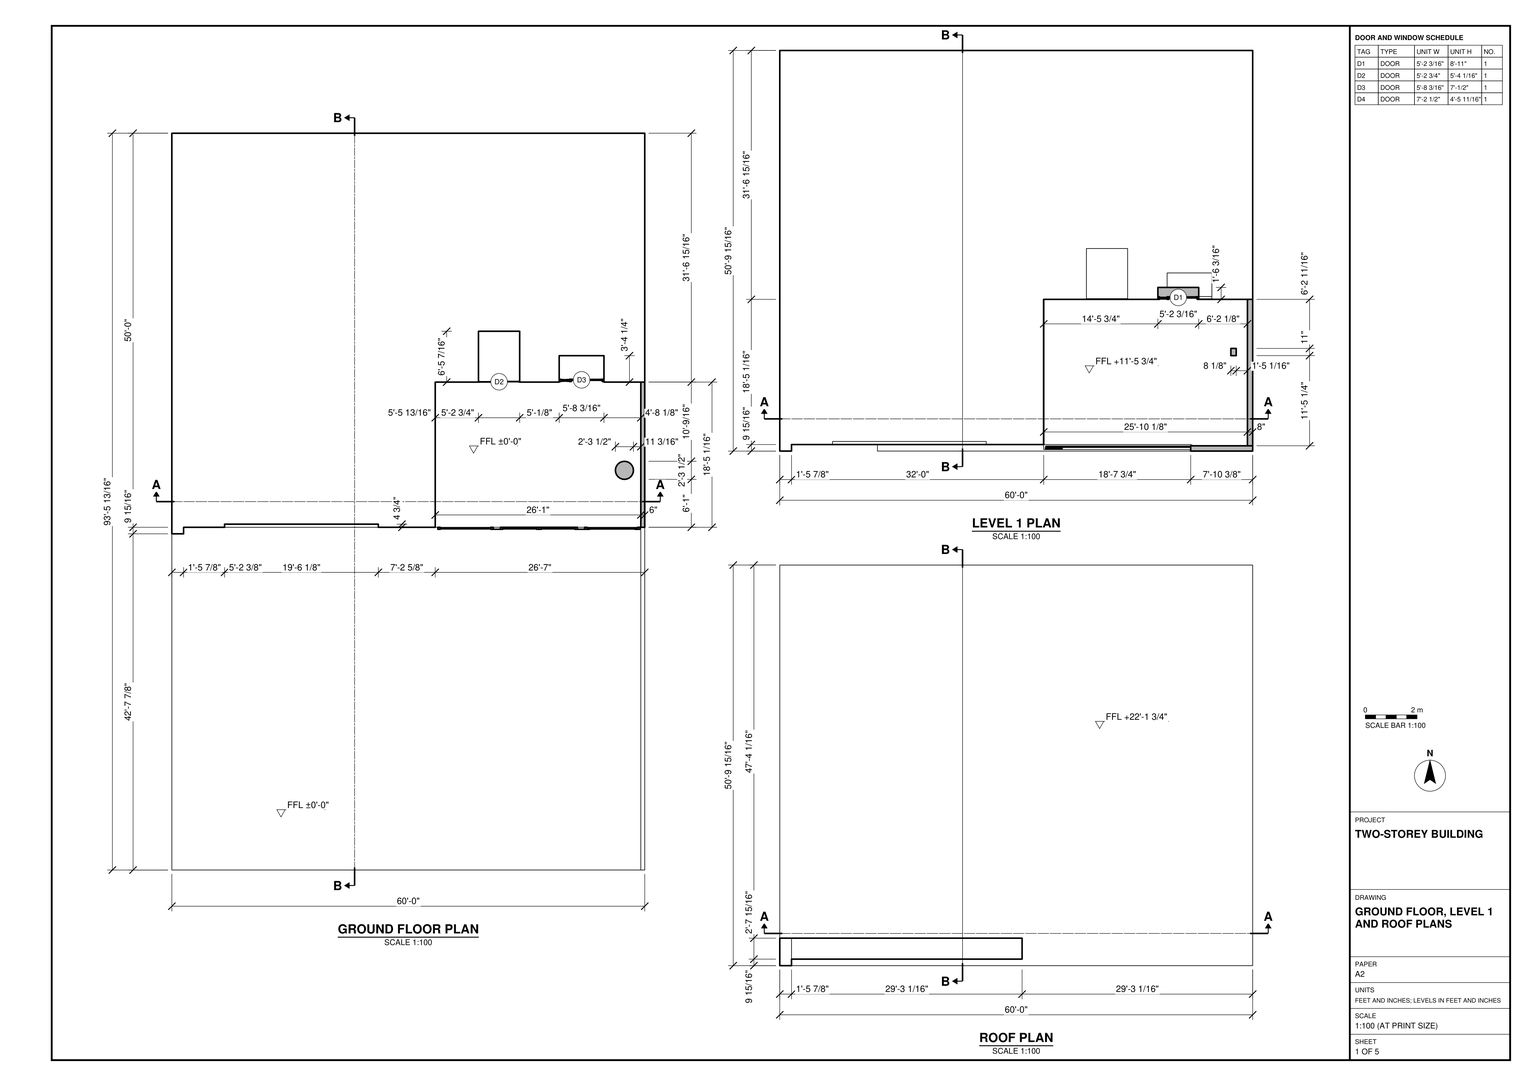
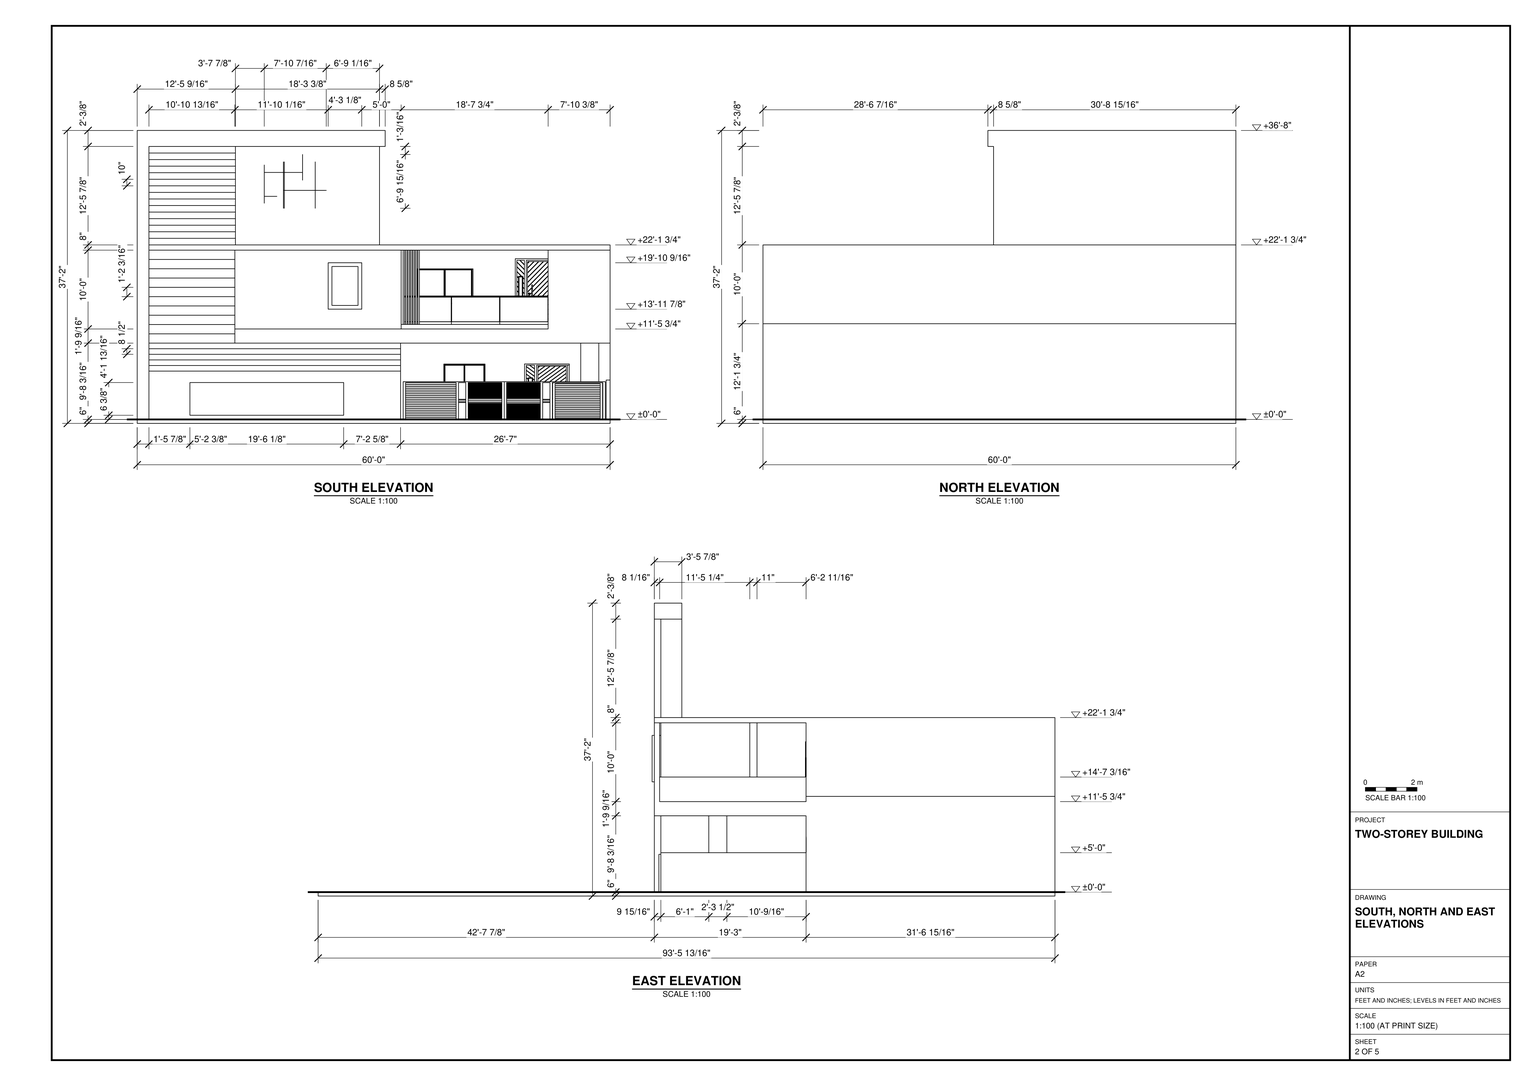
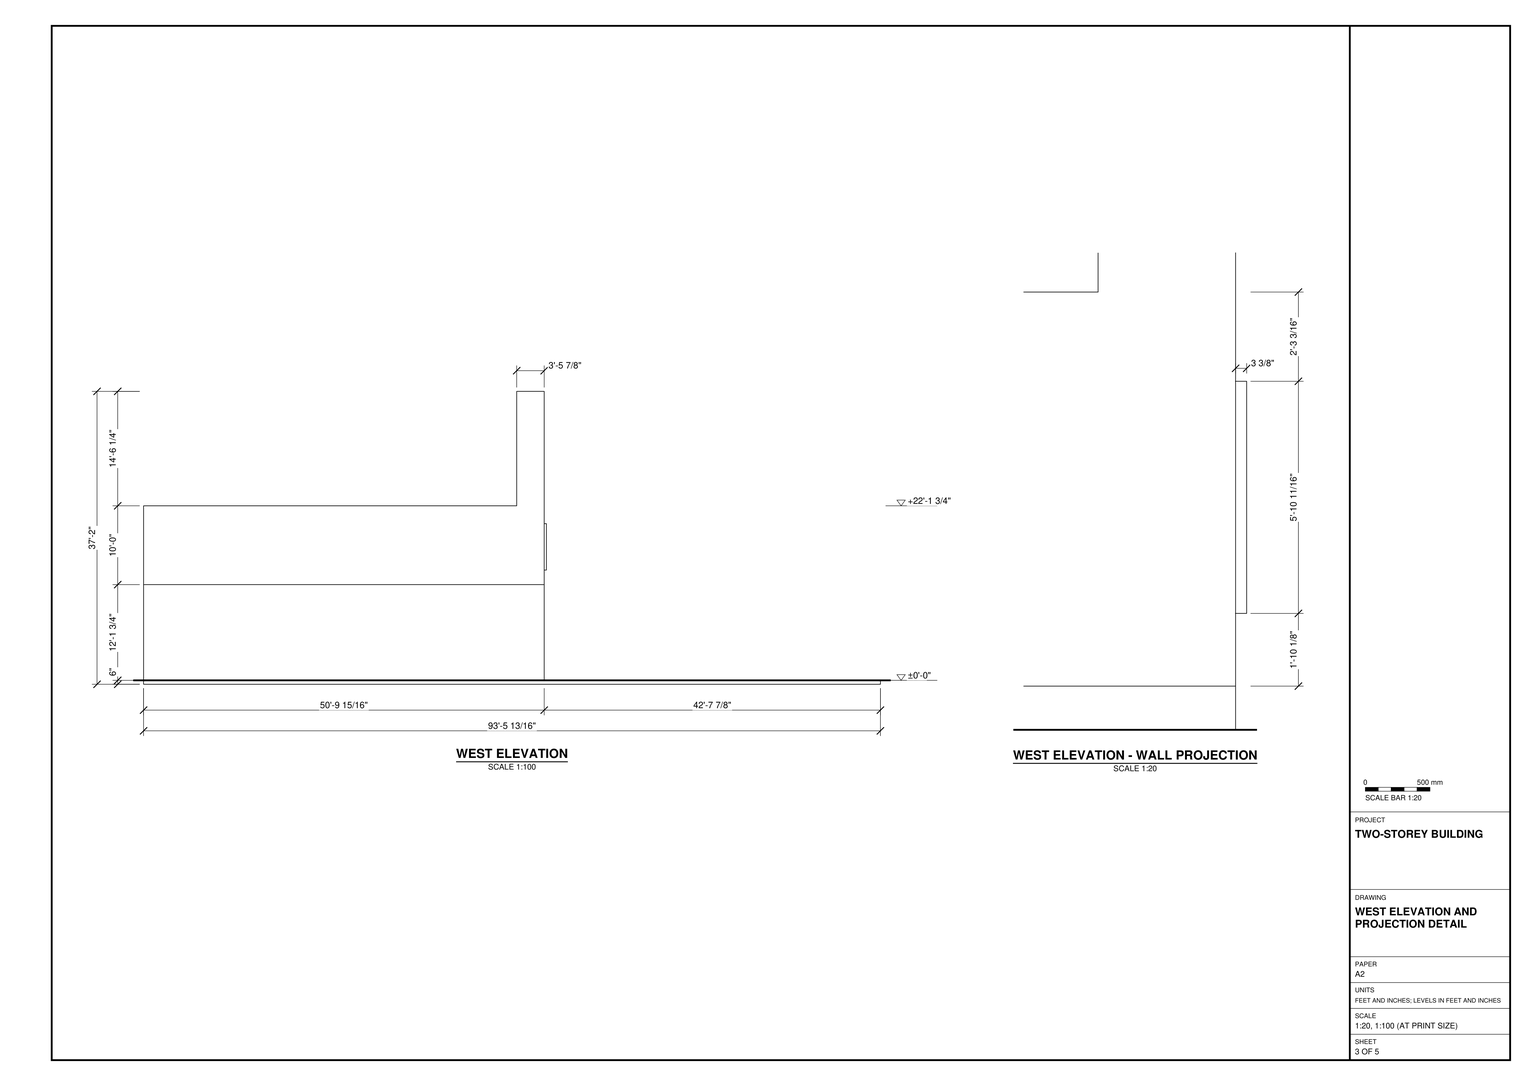
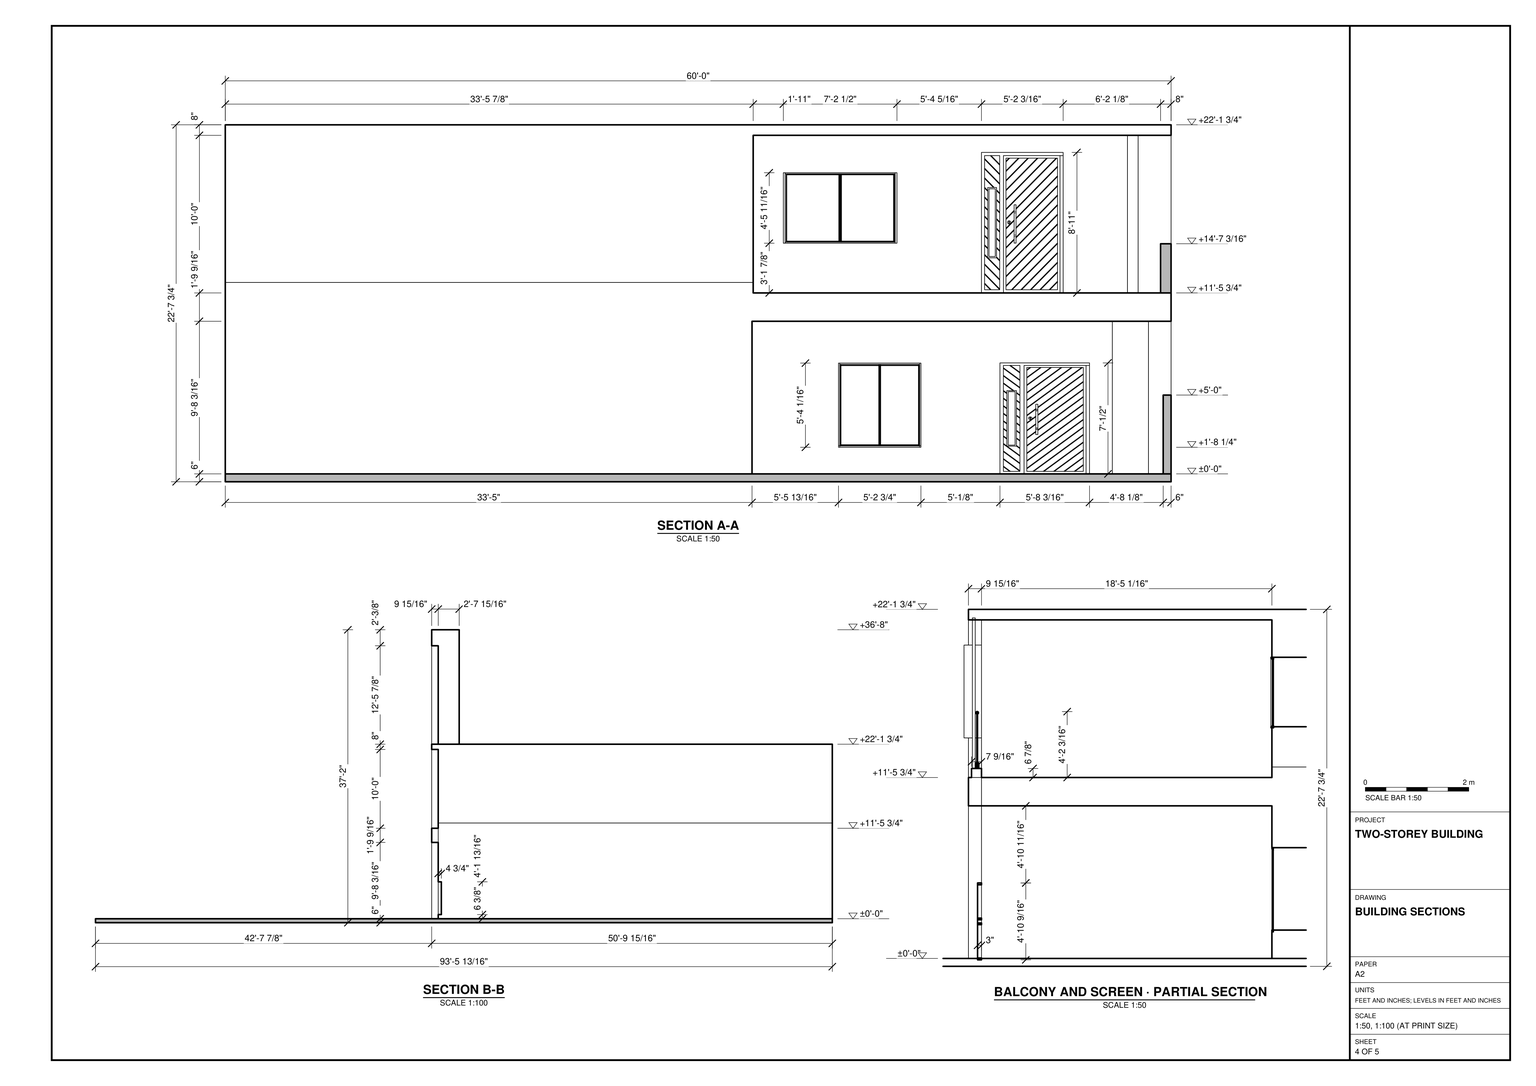
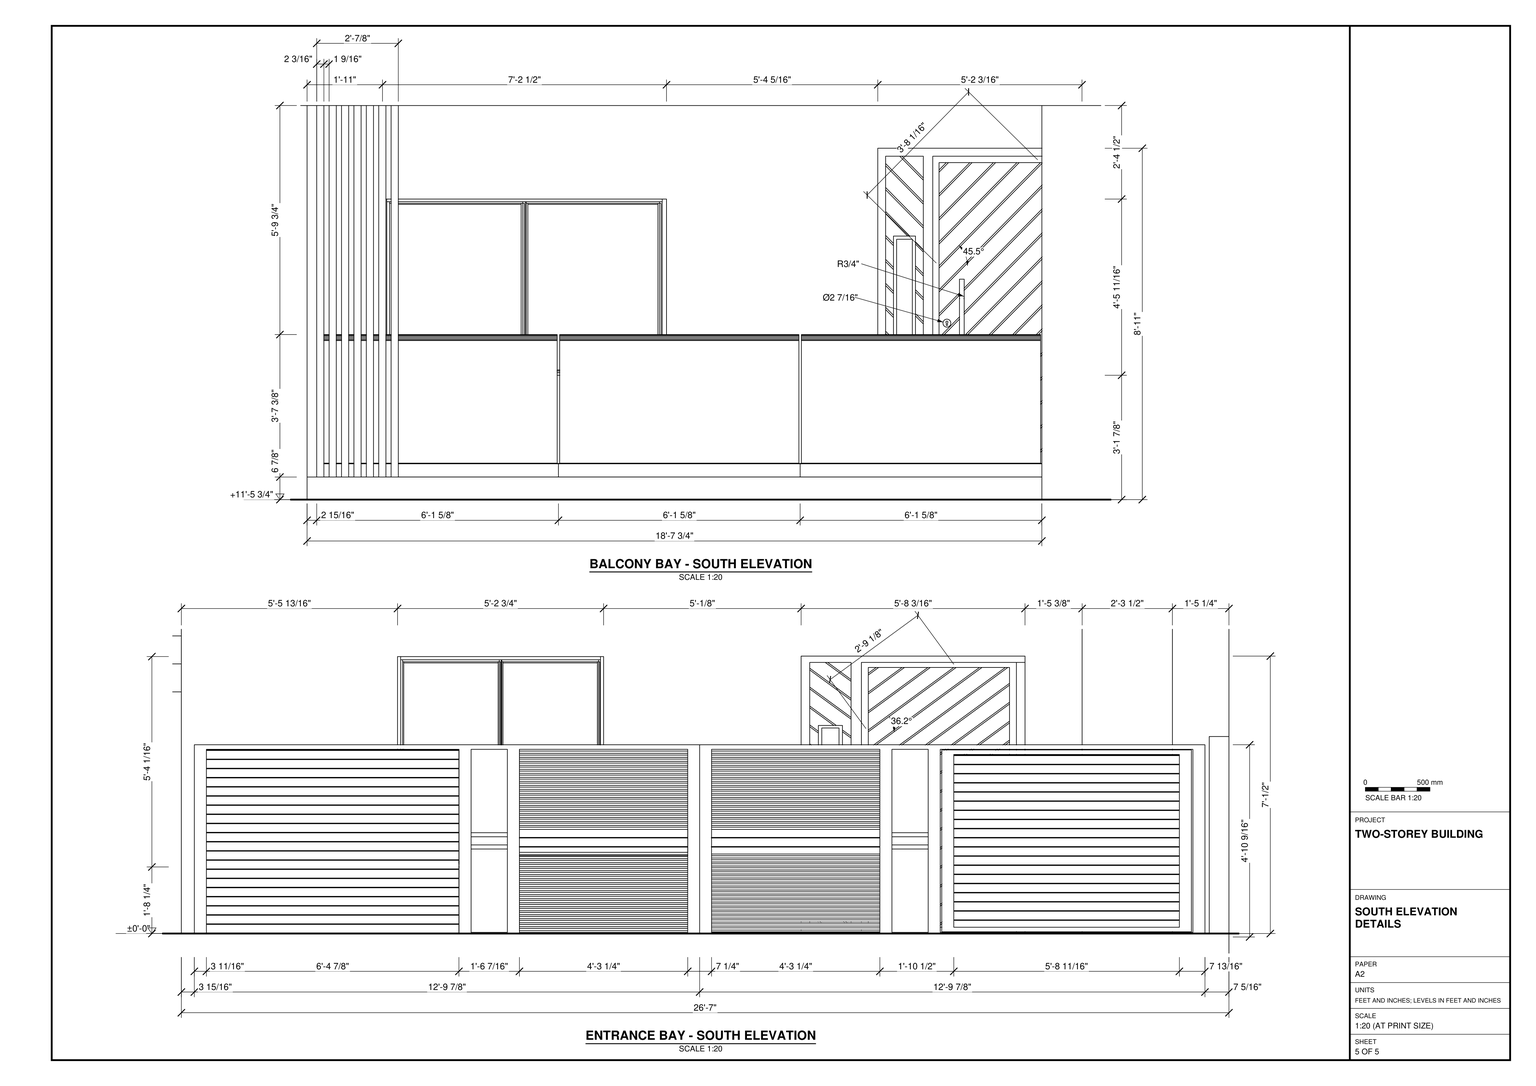
Build the two-storey building and its forecourt in SketchUp from task_files/diagram_01.pdf. Work in feet and inches. The complete model, including the forecourt slab, is 60'-0" wide, 93'-5 13/16" deep and 37'-2" high. Set the ground floor at ±0'-0", the upper floor at +11'-5 3/4" and the flat roof at +22'-1 3/4".

Place the building at the north end of the slab, with the forecourt facing the south elevation. Use the plans for wall thicknesses, slab edges, supports and door positions. On the east side of the south frontage, model the recessed ground-floor bay with its gate and side panels. Form the balcony directly above it, including the glass railing and the vertical screen at its west edge. On the west side of the frontage, reproduce the horizontal bands, the raised wall with its projecting cap, and the shallow framed wall projection shown in elevation and detail.

Keep shell elements such as walls, slabs and roof, and each furniture or joinery piece shown, in separate groups or components. Use components for repeated parts. Decor and loose items may be represented by any suitable library components. Save one SketchUp model as output_files/two_storey_building_with_a_gated_bay_and_balcony.skp.

# SketchUp Ruby script. Lengths in inches.
U = 1.inch
M = Sketchup.active_model
def pt(a) = Geom::Point3d.new(a.map { |v| v * U })
def face(e, loops, mat)
  f = e.add_face(loops[0].map { |a| pt(a) })
  loops[1..].each { |l| e.add_face(l.map { |a| pt(a) }).erase! }
  f.material = f.back_material = mat if mat
  f
end
# faces: each face lists its corners as indices into pts; further lists are holes
def faces(e, pts, list, mat = nil) = list.each { |f| face(e, (f[0].is_a?(Array) ? f : [f]).map { |l| l.map { |i| pts[i] } }, mat) }
# xy, xz, yz: faces in a plane at the given z, y or x. An outline is a flat list of corners, or four numbers for a rectangle; further outlines are holes
def ring(l) = l.size == 4 ? [[l[0], l[1]], [l[2], l[1]], [l[2], l[3]], [l[0], l[3]]] : l.each_slice(2).to_a
def flat(e, list, mat, &to3) = list.each { |f| face(e, (f[0].is_a?(Array) ? f : [f]).map { |l| ring(l).map { |u, v| to3.(u, v) } }, mat) }
def xy(e, z, list, mat = nil) = flat(e, list, mat) { |x, y| [x, y, z] }
def xz(e, y, list, mat = nil) = flat(e, list, mat) { |x, z| [x, y, z] }
def yz(e, x, list, mat = nil) = flat(e, list, mat) { |y, z| [x, y, z] }
def lines(e, pts, list) = list.each { |a, b| e.add_line(pt(pts[a]), pt(pts[b])) }
# prism: a flat outline (further loops are holes) pulled along v
def prism(e, loops, v, mat = nil)
  f = face(e, loops, mat); d = Geom::Vector3d.new(v.map { |x| x * U })
  f.pushpull(f.normal.samedirection?(d) ? d.length : -d.length)
end
def box(e, o, s, mat = nil) = prism(e, [[o, [o[0] + s[0], o[1], o[2]], [o[0] + s[0], o[1] + s[1], o[2]], [o[0], o[1] + s[1], o[2]]]], [0, 0, s[2]], mat)
def at(x, y, z, deg = 0) = Geom::Transformation.translation(pt([x, y, z])) * Geom::Transformation.rotation(ORIGIN, Z_AXIS, deg.degrees)
def axes(o, x, y, z) = Geom::Transformation.new([*x, 0, *y, 0, *z, 0, *pt(o).to_a, 1])
def part(name) = M.definitions.add(name)
# library, detail: a bought-in or finely detailed component or shape, given as its bounding box
def library(name, o, s) = part(name).tap { |d| box(d.entities, o, s) }
def detail(e, o, s) = box(e.add_group.entities, o, s)
def put(e, d, t, mat = nil) = e.add_instance(d, t).tap { |i| i.material = mat if mat }
def group(e, t, mat = nil) = e.add_group.tap { |g| g.transformation = t; g.material = mat if mat }.entities
root = M.entities
M.materials.add("Glass_Tinted_Gray").color = [0, 0, 0]
M.materials["Glass_Tinted_Gray"].alpha = 0.125
M.materials.add("[0134_DimGray]").color = [105, 105, 105]
M.materials.add("[0135_DarkGray]").color = [81, 81, 81]
M.materials.add("[Mirror 02]").color = [229, 229, 229]
M.materials.add("[Steel Brushed Stainless]1").color = [183, 187, 190]
M.materials.add("[Terrazzo Light Blue]").color = [196, 214, 227]
M.materials.add("[Wood Square Tile 01]").color = [164, 91, 44]
M.materials.add("[Wood Veneer 01]2").color = [120, 70, 37]
c1 = library("Glass Railings(black Handrails)",[-57.04,-132.55,0],[169.29,2.52,28.17])
c2 = part("PENTEK_RP Fineline 50S_Sliding_DoorCase_E1")
box(c2.entities,[0,0,0],[1.51,3.66,99.27],"[0135_DarkGray]")
c3 = part("PENTEK_RP Fineline 50S_SlidingDooe_Case_E2")
box(c3.entities,[0,0,0],[96.25,3.66,1.51],"[0135_DarkGray]")
c4 = part("pentek_RP Fineline 50S_SlidingDoor_Case")
put(c4.entities,c2,at(97.76,0,0))
put(c4.entities,c3,at(1.51,0,0))
put(c4.entities,c2,at(0,0,0))
put(c4.entities,c3,at(1.51,0,97.76))
c5 = part("PENTEK_RP Fineline 50S_SlidingDoor_GlazingBead_2")
box(c5.entities,[0,0,0],[0.56,0.59,94.39],"[0135_DarkGray]")
c6 = part("PENTEK_RP Fineline 50S_SlidingDoor_Glass")
box(c6.entities,[0,0,0],[46.58,0.16,94.39],"Glass_Tinted_Gray")
c7 = part("PENTEK_RP Fineline 50S_SlidingDoor_GlazingBead")
box(c7.entities,[0,0,0],[45.47,0.59,0.56],"[0135_DarkGray]")
c8 = part("PENTEK_RP Fineline 50S_SlidingDoor_Leaf_E1")
xy(c8.entities,0,[[0,0,0.93,1.97],[0.93,1.57,1.49,1.97]],"[0135_DarkGray]")
xy(c8.entities,96.25,[[0,0,0.93,0,0.93,1.57,1.49,1.57,1.49,1.97,0,1.97]],"[0135_DarkGray]")
xz(c8.entities,0,[[0,0,0.93,96.25]],"[0135_DarkGray]")
xz(c8.entities,1.57,[[0.93,0,1.49,95.32],[0.93,95.32,1.49,96.25]],"[0135_DarkGray]")
xz(c8.entities,1.97,[[0,0,1.49,96.25]],"[0135_DarkGray]")
yz(c8.entities,0,[[0,0,1.97,96.25]],"[0135_DarkGray]")
yz(c8.entities,0.93,[[0,0,1.57,0.93],[0,0.93,1.57,95.32],[0,95.32,1.57,96.25]],"[0135_DarkGray]")
yz(c8.entities,1.49,[[1.57,0,1.97,95.32],[1.57,95.32,1.97,96.25]],"[0135_DarkGray]")
c9 = part("PENTEK_RP Fineline 50S_SlidingDoor_Leaf_E2")
xy(c9.entities,0,[[0,0,0,1.57,0.56,1.57,0.56,1.97,46.02,1.97,46.02,1.57,46.58,1.57,46.58,0]],"[0135_DarkGray]")
xy(c9.entities,0.93,[[0,0,46.58,1.57]],"[0135_DarkGray]")
xy(c9.entities,1.49,[[0.56,1.57,46.02,1.97]],"[0135_DarkGray]")
xz(c9.entities,0,[[0,0,46.58,0.93]],"[0135_DarkGray]")
xz(c9.entities,1.57,[[0,0,0.56,0.93],[46.02,0,46.58,0.93],[0.56,0.93,46.02,1.49]],"[0135_DarkGray]")
xz(c9.entities,1.97,[[0.56,0,46.02,1.49]],"[0135_DarkGray]")
yz(c9.entities,0,[[0,0,1.57,0.93]],"[0135_DarkGray]")
yz(c9.entities,0.56,[[1.57,0,1.97,0.93],[1.57,0.93,1.97,1.49]],"[0135_DarkGray]")
yz(c9.entities,46.02,[[1.57,0,1.97,0.93],[1.57,0.93,1.97,1.49]],"[0135_DarkGray]")
yz(c9.entities,46.58,[[0,0,1.57,0.93]],"[0135_DarkGray]")
c10 = part("PENTEK_RP Fineline S_SlidingDoor_Leaf1")
put(c10.entities,c5,at(0.93,0,0.93))
put(c10.entities,c5,at(46.96,0,0.93))
put(c10.entities,c6,at(1.49,1.42,0.93))
put(c10.entities,c7,at(1.49,0,0.93))
put(c10.entities,c6,at(1.49,0.59,0.93),"[Terrazzo Light Blue]")
put(c10.entities,c8,at(0,0,0))
put(c10.entities,c8,axes([48.44,0,0],[-1,0,0],[0,1,0],[0,0,1]))
put(c10.entities,c9,axes([0.93,0,96.25],[1,0,0],[0,1,0],[0,0,-1]))
put(c10.entities,c9,at(0.93,0,0))
put(c10.entities,c7,at(1.49,0,94.77))
c11 = part("PENTEK_RP Fineline 50S_SlidingDoor_Leaf2")
put(c11.entities,c6,at(1.49,1.42,0.93))
put(c11.entities,c7,at(1.49,0,94.77))
put(c11.entities,c5,at(46.96,0,0.93))
put(c11.entities,c6,at(1.49,0.59,0.93),"[Mirror 02]")
put(c11.entities,c5,at(0.93,0,0.93))
put(c11.entities,c8,at(0,0,0))
put(c11.entities,c8,axes([48.44,0,0],[-1,0,0],[0,1,0],[0,0,1]))
put(c11.entities,c7,at(1.49,0,0.93))
put(c11.entities,c9,axes([0.93,0,96.25],[1,0,0],[0,1,0],[0,0,-1]))
put(c11.entities,c9,at(0.93,0,0))
c12 = part("PENTEK - Slimmest Steel Sliding Door / Window\#1")
put(c12.entities,c4,at(0,-1.88,-0.09))
put(c12.entities,c10,at(1.51,-2.27,1.42))
put(c12.entities,c11,at(49.32,-0.3,1.42))
c13 = library("Door 7",[39.1,8.76,0],[51.18,7.87,86.61])
c14 = part("Gate board")
g1 = group(c14.entities,at(0,0,0))
box(g1,[-1.63,0,-0.61],[45.72,0.75,5.61],"[Wood Veneer 01]2")
c15 = part("Gate board \#1")
g2 = group(c15.entities,at(0,0,0))
box(g2,[12.91,0,-0.61],[31.18,0.75,5.61],"[Wood Veneer 01]2")
c16 = part("Gate slat")
box(c16.entities,[-30,-0.5,-0.88],[29.34,1,1.38])
c17 = part("Slatted gate panel")
put(c17.entities,c16,axes([28.6,0,4.125],[0.95345,0,0],[0,1,0],[0,0,0.71186]),"[Steel Brushed Stainless]1")
put(c17.entities,c16,axes([28.6,0,11.125],[0.95345,0,0],[0,1,0],[0,0,0.71186]),"[Steel Brushed Stainless]1")
put(c17.entities,c16,axes([28.6,0,32.125],[0.95345,0,0],[0,1,0],[0,0,0.71186]),"[Steel Brushed Stainless]1")
put(c17.entities,c16,axes([28.6,0,14.625],[0.95345,0,0],[0,1,0],[0,0,0.71186]),"[Steel Brushed Stainless]1")
put(c17.entities,c16,axes([28.6,0,28.625],[0.95345,0,0],[0,1,0],[0,0,0.71186]),"[Steel Brushed Stainless]1")
put(c17.entities,c16,axes([28.6,0,0.625],[0.95345,0,0],[0,1,0],[0,0,0.71186]),"[Steel Brushed Stainless]1")
put(c17.entities,c16,axes([28.6,0,7.625],[0.95345,0,0],[0,1,0],[0,0,0.71186]),"[Steel Brushed Stainless]1")
put(c17.entities,c16,axes([28.6,0,12.875],[0.95345,0,0],[0,1,0],[0,0,0.71186]),"[Steel Brushed Stainless]1")
put(c17.entities,c16,axes([28.6,0,5.875],[0.95345,0,0],[0,1,0],[0,0,0.71186]),"[Steel Brushed Stainless]1")
put(c17.entities,c16,axes([28.6,0,25.125],[0.95345,0,0],[0,1,0],[0,0,0.71186]),"[Steel Brushed Stainless]1")
put(c17.entities,c16,axes([28.6,0,18.125],[0.95345,0,0],[0,1,0],[0,0,0.71186]),"[Steel Brushed Stainless]1")
put(c17.entities,c16,axes([28.6,0,23.375],[0.95345,0,0],[0,1,0],[0,0,0.71186]),"[Steel Brushed Stainless]1")
put(c17.entities,c16,axes([28.6,0,26.875],[0.95345,0,0],[0,1,0],[0,0,0.71186]),"[Steel Brushed Stainless]1")
put(c17.entities,c16,axes([28.6,0,16.375],[0.95345,0,0],[0,1,0],[0,0,0.71186]),"[Steel Brushed Stainless]1")
put(c17.entities,c16,axes([28.6,0,30.375],[0.95345,0,0],[0,1,0],[0,0,0.71186]),"[Steel Brushed Stainless]1")
put(c17.entities,c16,axes([28.6,0,21.625],[0.95345,0,0],[0,1,0],[0,0,0.71186]),"[Steel Brushed Stainless]1")
put(c17.entities,c16,axes([28.6,0,19.875],[0.95345,0,0],[0,1,0],[0,0,0.71186]),"[Steel Brushed Stainless]1")
put(c17.entities,c16,axes([28.6,0,2.375],[0.95345,0,0],[0,1,0],[0,0,0.71186]),"[Steel Brushed Stainless]1")
put(c17.entities,c16,axes([28.6,0,9.375],[0.95345,0,0],[0,1,0],[0,0,0.71186]),"[Steel Brushed Stainless]1")
put(c17.entities,c16,axes([28.6,0,33.875],[0.95345,0,0],[0,1,0],[0,0,0.71186]),"[Steel Brushed Stainless]1")
c18 = part("gatehalf\#2")
put(c18.entities,c14,axes([45.23,2.15,109.78],[1,0,0],[0,0.93969,0.48046],[0,-0.24347,0.93969]))
put(c18.entities,c15,axes([-10.77,2.15,61.69],[1,0,0],[0,0.93969,0.48046],[0,-0.24347,0.93969]))
put(c18.entities,c17,axes([2.16,2.5,2.82],[1.08929,0,0],[0,1,0],[0,0,1.40476]))
put(c18.entities,c17,axes([2.16,0.5,3.88],[1.08929,0,0],[0,1,0],[0,0,1.40476]))
put(c18.entities,c14,axes([45.23,2.15,104.16],[1,0,0],[0,0.93969,0.48046],[0,-0.24347,0.93969]))
put(c18.entities,c14,axes([45.23,2.15,98.54],[1,0,0],[0,0.93969,0.48046],[0,-0.24347,0.93969]))
put(c18.entities,c14,axes([45.23,2.15,92.92],[1,0,0],[0,0.93969,0.48046],[0,-0.24347,0.93969]))
put(c18.entities,c14,axes([45.23,2.15,87.3],[1,0,0],[0,0.93969,0.48046],[0,-0.24347,0.93969]))
put(c18.entities,c14,axes([45.23,2.15,81.68],[1,0,0],[0,0.93969,0.48046],[0,-0.24347,0.93969]))
put(c18.entities,c14,axes([45.23,2.15,76.0625],[1,0,0],[0,0.93969,0.48046],[0,-0.24347,0.93969]))
put(c18.entities,c14,axes([45.23,2.15,70.44],[1,0,0],[0,0.93969,0.48046],[0,-0.24347,0.93969]))
put(c18.entities,c14,axes([45.23,2.15,64.83],[1,0,0],[0,0.93969,0.48046],[0,-0.24347,0.93969]))
put(c18.entities,c14,axes([45.23,2.15,59.21],[1,0,0],[0,0.93969,0.48046],[0,-0.24347,0.93969]))
put(c18.entities,c14,axes([45.23,2.15,53.59],[1,0,0],[0,0.93969,0.48046],[0,-0.24347,0.93969]))
put(c18.entities,c14,axes([45.23,2.15,47.97],[1,0,0],[0,0.93969,0.48046],[0,-0.24347,0.93969]))
put(c18.entities,c14,axes([45.23,2.15,42.35],[1,0,0],[0,0.93969,0.48046],[0,-0.24347,0.93969]))
put(c18.entities,c14,axes([45.23,2.15,36.73],[1,0,0],[0,0.93969,0.48046],[0,-0.24347,0.93969]))
put(c18.entities,c14,axes([45.23,2.15,31.11],[1,0,0],[0,0.93969,0.48046],[0,-0.24347,0.93969]))
put(c18.entities,c14,axes([45.23,2.15,25.49],[1,0,0],[0,0.93969,0.48046],[0,-0.24347,0.93969]))
put(c18.entities,c14,axes([45.23,2.15,19.875],[1,0,0],[0,0.93969,0.48046],[0,-0.24347,0.93969]))
put(c18.entities,c14,axes([45.23,2.15,14.25],[1,0,0],[0,0.93969,0.48046],[0,-0.24347,0.93969]))
put(c18.entities,c14,axes([45.23,2.15,8.64],[1,0,0],[0,0.93969,0.48046],[0,-0.24347,0.93969]))
put(c18.entities,c14,axes([45.23,2.15,3.02],[1,0,0],[0,0.93969,0.48046],[0,-0.24347,0.93969]))
put(c18.entities,c15,axes([-10.77,2.15,56.07],[1,0,0],[0,0.93969,0.48046],[0,-0.24347,0.93969]))
put(c18.entities,c15,axes([-10.77,2.15,50.45],[1,0,0],[0,0.93969,0.48046],[0,-0.24347,0.93969]))
g3 = group(c18.entities,at(0,0,0))
prism(g3,[[[0,3,118],[91.5,3,118],[91.5,3,0],[0,3,0]],[[43.57,3,115.18],[43.57,3,2.3],[89.32,3,2.3],[89.32,3,115.18]],[[32.64,3,115.18],[2.16,3,115.18],[2.16,3,2.82],[32.64,3,2.82]],[[34.82,3,2.82],[41.39,3,2.82],[41.39,3,54],[34.82,3,54]],[[34.82,3,115.18],[34.82,3,64],[41.39,3,64],[41.39,3,115.18]],[[41.39,3,56.5],[41.39,3,61.5],[34.82,3,61.5],[34.82,3,56.5]]],[0,-3,0],"[Steel Brushed Stainless]1")
g4 = group(c18.entities,at(2.16,0,66.04))
put(g4,c17,axes([0,0.5,0],[1.08929,0,0],[0,1,0],[0,0,1.40476]))
put(g4,c17,axes([0,2.5,1.05],[1.08929,0,0],[0,1,0],[0,0,1.40476]))
c19 = part("Timber board")
box(c19.entities,[0,0,0],[37.5,0.75,4],"[Wood Veneer 01]2")
c20 = part("gatehalf\#1")
put(c20.entities,c15,axes([45.55,2.15,56.07],[-1,0,0],[0,0.93969,0.48046],[0,-0.24347,0.93969]))
put(c20.entities,c15,axes([45.55,2.15,61.69],[-1,0,0],[0,0.93969,0.48046],[0,-0.24347,0.93969]))
put(c20.entities,c15,axes([45.55,2.15,50.45],[-1,0,0],[0,0.93969,0.48046],[0,-0.24347,0.93969]))
g5 = group(c20.entities,at(0,0,0))
prism(g5,[[[0,3,118],[91.5,3,118],[91.5,3,0],[0,3,0]],[[43.57,3,115.18],[43.57,3,2.82],[89.32,3,2.82],[89.32,3,115.18]],[[32.64,3,115.18],[2.16,3,115.18],[2.16,3,2.82],[32.64,3,2.82]],[[34.82,3,2.82],[41.39,3,2.82],[41.39,3,54],[34.82,3,54]],[[34.82,3,115.18],[34.82,3,64],[41.39,3,64],[41.39,3,115.18]],[[41.39,3,56.5],[41.39,3,61.5],[34.82,3,61.5],[34.82,3,56.5]]],[0,-3,0],"[Steel Brushed Stainless]1")
g6 = group(c20.entities,at(42.96,0,3.18))
put(g6,c19,axes([3.0625,1.3,102.86],[1.08929,0,0],[0,0.93969,0.48046],[0,-0.34202,1.32004]))
put(g6,c19,axes([3.0625,1.3,97.24],[1.08929,0,0],[0,0.93969,0.48046],[0,-0.34202,1.32004]))
put(g6,c19,axes([3.0625,1.3,91.62],[1.08929,0,0],[0,0.93969,0.48046],[0,-0.34202,1.32004]))
put(g6,c19,axes([3.0625,1.3,86],[1.08929,0,0],[0,0.93969,0.48046],[0,-0.34202,1.32004]))
put(g6,c19,axes([3.0625,1.3,80.38],[1.08929,0,0],[0,0.93969,0.48046],[0,-0.34202,1.32004]))
put(g6,c19,axes([3.0625,1.3,74.76],[1.08929,0,0],[0,0.93969,0.48046],[0,-0.34202,1.32004]))
put(g6,c19,axes([3.0625,1.3,69.15],[1.08929,0,0],[0,0.93969,0.48046],[0,-0.34202,1.32004]))
put(g6,c19,axes([3.0625,1.3,63.53],[1.08929,0,0],[0,0.93969,0.48046],[0,-0.34202,1.32004]))
put(g6,c19,axes([3.0625,1.3,57.91],[1.08929,0,0],[0,0.93969,0.48046],[0,-0.34202,1.32004]))
put(g6,c19,axes([3.0625,1.3,52.29],[1.08929,0,0],[0,0.93969,0.48046],[0,-0.34202,1.32004]))
put(g6,c19,axes([3.0625,1.3,46.67],[1.08929,0,0],[0,0.93969,0.48046],[0,-0.34202,1.32004]))
put(g6,c19,axes([3.0625,1.3,41.05],[1.08929,0,0],[0,0.93969,0.48046],[0,-0.34202,1.32004]))
put(g6,c19,axes([3.0625,1.3,35.43],[1.08929,0,0],[0,0.93969,0.48046],[0,-0.34202,1.32004]))
put(g6,c19,axes([3.0625,1.3,29.8125],[1.08929,0,0],[0,0.93969,0.48046],[0,-0.34202,1.32004]))
put(g6,c19,axes([3.0625,1.3,24.19],[1.08929,0,0],[0,0.93969,0.48046],[0,-0.34202,1.32004]))
put(g6,c19,axes([3.0625,1.3,18.57],[1.08929,0,0],[0,0.93969,0.48046],[0,-0.34202,1.32004]))
put(g6,c19,axes([3.0625,1.3,12.96],[1.08929,0,0],[0,0.93969,0.48046],[0,-0.34202,1.32004]))
put(g6,c19,axes([3.0625,1.3,7.34],[1.08929,0,0],[0,0.93969,0.48046],[0,-0.34202,1.32004]))
put(g6,c19,axes([3.0625,1.3,1.72],[1.08929,0,0],[0,0.93969,0.48046],[0,-0.34202,1.32004]))
g7 = group(g6,at(0,0,0))
prism(g7,[[[0.89,2,111.65],[46.09,2,111.65],[46.09,2,0],[0.89,2,0]],[[43.91,2,2.81],[43.91,2,108.84],[3.0625,2,108.84],[3.0625,2,2.81]]],[0,-2,0],"[Steel Brushed Stainless]1")
g8 = group(c20.entities,at(32.64,0,66.04))
put(g8,c17,axes([0,0.5,0],[-1.08929,0,0],[0,1,0],[0,0,1.40476]))
put(g8,c17,axes([0,2.5,1.05],[-1.08929,0,0],[0,1,0],[0,0,1.40476]))
g9 = group(c20.entities,at(32.64,0,1.77))
put(g9,c17,axes([0,0.5,0],[-1.08929,0,0],[0,1,0],[0,0,1.40476]))
put(g9,c17,axes([0,2.5,1.05],[-1.08929,0,0],[0,1,0],[0,0,1.40476]))
c21 = part("MainGate_20210604Bskp")
g10 = group(c21.entities,at(229.23,747.46,0))
xz(g10,0,[[46.01,2.01,52.03,81.99],[115.97,2.01,121.99,81.99]],"[Steel Brushed Stainless]1")
put(g10,c18,axes([84,0,0],[-0.91803,0,0],[0,1,0],[0,0,0.71186]))
put(g10,c20,axes([84,0,0],[0.91803,0,0],[0,1,0],[0,0,0.71186]))
xy(root,-31.75,[[0,0,720,1121.8125]])
xy(root,-25.75,[[0,0,714,0,714,521.8125,17.875,521.8125,17.875,511.875,0,511.875],[714,0,720,521.8125],[0,511.875,17.875,511.875,17.875,521.8125,400.99,521.8125,400.99,742.875,589.73,742.875,589.73,783.125,657.9,783.125,657.9,742.875,720,742.875,720,1121.8125,0,1121.8125],[[400.99,521.8125,714,521.8125,714,742.875,657.9,742.875,657.9,783.125,589.73,783.125,589.73,742.875,400.99,742.875],[689.04,594.8,685.48,595.27,682.16,596.64,679.32,598.83,677.13,601.67,675.76,604.99,675.29,608.55,675.76,612.11,677.13,615.42,679.32,618.27,682.16,620.46,685.48,621.83,689.04,622.3,692.6,621.83,695.91,620.46,698.76,618.27,700.95,615.42,702.32,612.11,702.79,608.55,702.32,604.99,700.95,601.67,698.76,598.83,695.91,596.64,692.6,595.27]],[714,521.8125,720,742.875]])
xy(root,-19.38,[[80.25,521.8125,314.37,526.5625]])
xy(root,-4.16,[[466.83,742.875,529.58,820.3125]])
xy(root,30.43,[[80.25,521.8125,314.37,526.5625]])
xy(root,34.25,[[714,521.8125,720,742.875]])
xy(root,58.59,[[466.83,742.875,529.58,820.3125]])
xy(root,58.74,[[589.73,742.875,657.9,783.125]])
xy(root,90.4375,[[[148.69,511.875,148.69,521.8125,400.99,521.8125,400.99,742.875,720,742.875,720,511.875],[689.04,594.8,692.6,595.27,695.91,596.64,698.76,598.83,700.95,601.67,702.32,604.99,702.79,608.55,702.32,612.11,700.95,615.42,698.76,618.27,695.91,620.46,692.6,621.83,689.04,622.3,685.48,621.83,682.16,620.46,679.32,618.27,677.13,615.42,675.76,612.11,675.29,608.55,675.76,604.99,677.13,601.67,679.32,598.83,682.16,596.64,685.48,595.27]]])
xy(root,112,[[148.69,511.875,625.625,511.875,625.625,514.22,401.88,514.22,401.88,521.8125,148.69,521.8125],[[625.625,519.9375,712,519.9375,712,742.875,637.84,742.875,637.84,761.0625,575.66,761.0625,575.66,742.875,401.88,742.875,401.88,521.8125,625.625,521.8125],[686.79,657.2,694.92,668.2]],[712,519.9375,720,742.875]])
xy(root,118.875,[[[401.88,514.22,625.625,521.8125],[404.8125,514.85,407,517.04],[408.59,514.85,410.78,517.04],[412.37,514.85,414.55,517.04],[416.14,514.85,418.33,517.04],[419.92,514.85,422.11,517.04],[423.7,514.85,425.89,517.04],[427.47,514.85,429.66,517.04]]])
xy(root,142.14,[[290.78,508.5,341.9,521.8125]])
xy(root,147.83,[[296.47,508.5,336.21,521.8125]])
xy(root,149.4375,[[712,519.9375,720,742.875]])
xy(root,150.65,[[424.85,742.875,510.4,827.9375]])
xy(root,203.52,[[424.85,742.875,510.4,827.9375]])
xy(root,207.13,[[296.47,508.5,336.21,521.8125]])
xy(root,212.83,[[290.78,508.5,341.9,521.8125]])
xy(root,219,[[575.66,742.875,637.84,761.0625]])
xy(root,232,[[[17.875,511.875,17.875,521.8125,401.88,521.8125,401.88,742.875,720,742.875,720,519.9375,625.625,519.9375,625.625,511.875],[686.79,657.2,694.92,668.2],[404.8125,514.85,407,517.04],[412.37,514.85,414.55,517.04],[419.92,514.85,422.11,517.04],[423.7,514.85,425.89,517.04],[427.47,514.85,429.66,517.04]]])
xy(root,232.25,[[416.14,514.85,418.33,517.04]])
xy(root,233.5,[[408.59,514.85,410.78,517.04]])
xy(root,240,[[17.875,511.875,720,511.875,720,1121.8125,0,1121.8125,0,553.75,368.9375,553.75,368.9375,521.8125,17.875,521.8125],[17.875,521.8125,368.9375,553.75]])
xy(root,389.89,[[17.875,511.875,17.875,521.8125,368.9375,521.8125,368.9375,553.75,377.5625,553.75,377.5625,511.875]])
xy(root,414.25,[[0,511.875,377.5625,553.75]])
xz(root,0,[[0,-31.75,720,-25.75]])
xz(root,508.5,[[[290.78,142.14,341.9,212.83],[296.47,147.83,336.21,207.13]]])
xz(root,511.875,[[0,-25.75,17.875,-25.75,17.875,389.89,377.5625,389.89,377.5625,414.25,0,414.25],[148.69,90.4375,720,90.4375,720,232,625.625,232,625.625,112,148.69,112],[17.875,232,720,240]])
xz(root,514.22,[[401.88,112,625.625,118.875]])
xz(root,514.85,[[404.8125,118.875,407,232],[408.59,118.875,410.78,233.5],[412.37,118.875,414.55,232],[416.14,118.875,418.33,232.25],[419.92,118.875,422.11,232],
  [423.7,118.875,425.89,232],[427.47,118.875,429.66,232]])
xz(root,517.04,[[404.8125,118.875,407,232],[408.59,118.875,410.78,233.5],[412.37,118.875,414.55,232],[416.14,118.875,418.33,232.25],[419.92,118.875,422.11,232],
  [423.7,118.875,425.89,232],[427.47,118.875,429.66,232]])
xz(root,519.9375,[[625.625,112,625.625,232,720,232,720,149.4375,712,149.4375,712,112],[712,112,720,149.4375]])
xz(root,521.8125,[[[17.875,-25.75,400.99,47.84],[80.25,-19.38,314.37,30.43]],[714,-25.75,720,34.25],[[148.69,112,401.88,232],[290.78,142.14,341.9,212.83]],[401.88,112,625.625,118.875],[296.47,147.83,336.21,207.13]])
xz(root,521.8125,[[[149.56,240,368.9375,389.89],[222.62,323.03,223.99,350.3125]],[222.62,323.03,223.99,350.3125]],"[0134_DimGray]")
xz(root,521.8125,[[17.875,47.84,400.99,56.36],[17.875,56.36,400.99,64.88],[17.875,64.88,400.99,73.4],[17.875,73.4,400.99,81.92],[17.875,81.92,400.99,90.4375],
  [17.875,90.4375,148.69,104.59],[17.875,104.59,148.69,118.75],[17.875,118.75,148.69,132.91],[17.875,132.91,148.69,147.0625],[17.875,147.0625,148.69,161.22],
  [17.875,161.22,148.69,175.375],[17.875,175.375,148.69,189.53],[17.875,189.53,148.69,203.6875],[17.875,203.6875,148.69,217.84],[17.875,217.84,148.69,232],
  [17.875,240,149.56,249.99],[17.875,249.99,149.56,259.98],[17.875,259.98,149.56,269.98],[17.875,269.98,149.56,279.97],[17.875,279.97,149.56,289.96],
  [17.875,289.96,149.56,299.95],[17.875,299.95,149.56,309.95],[17.875,309.95,149.56,319.94],[17.875,319.94,149.56,329.93],[17.875,329.93,149.56,339.92],
  [17.875,339.92,149.56,349.92],[17.875,349.92,149.56,359.91],[17.875,359.91,149.56,369.9],[17.875,369.9,149.56,379.89],[17.875,379.89,149.56,389.89]],"[Wood Square Tile 01]")
xz(root,526.5625,[[80.25,-19.38,314.37,30.43]])
xz(root,553.75,[[0,240,0,414.25,377.5625,414.25,377.5625,389.89,368.9375,389.89,368.9375,240]])
xz(root,657.2,[[686.79,112,694.92,232]])
xz(root,668.2,[[686.79,112,694.92,232]])
xz(root,742.875,[[[400.99,-25.75,589.73,-25.75,589.73,58.74,657.9,58.74,657.9,-25.75,714,-25.75,714,34.25,720,34.25,720,90.4375,400.99,90.4375],[466.83,-4.16,529.58,58.59]],[714,-25.75,720,34.25],[[401.88,112,575.66,112,575.66,219,637.84,219,637.84,112,712,112,712,149.4375,720,149.4375,720,232,401.88,232],[424.85,150.65,510.4,203.52]],[712,112,720,149.4375]])
xz(root,761.0625,[[575.66,112,637.84,219]])
xz(root,783.125,[[589.73,-25.75,657.9,58.74]])
xz(root,820.3125,[[466.83,-4.16,529.58,58.59]])
xz(root,827.9375,[[424.85,150.65,510.4,203.52]])
xz(root,1121.8125,[[0,-31.75,720,-25.75],[0,-25.75,720,120],[0,120,720,240]])
yz(root,0,[[0,-31.75,1121.8125,-25.75],[511.875,-25.75,1121.8125,120],[511.875,120,511.875,414.25,553.75,414.25,553.75,240,1121.8125,240,1121.8125,120]])
yz(root,17.875,[[511.875,-25.75,521.8125,232],[511.875,240,521.8125,389.89]])
yz(root,80.25,[[521.8125,-19.38,526.5625,30.43]])
yz(root,148.69,[[511.875,90.4375,521.8125,112]])
yz(root,290.78,[[508.5,142.14,521.8125,212.83]])
yz(root,296.47,[[508.5,147.83,521.8125,207.13]])
yz(root,314.37,[[521.8125,-19.38,526.5625,30.43]])
yz(root,336.21,[[508.5,147.83,521.8125,207.13]])
yz(root,341.9,[[508.5,142.14,521.8125,212.83]])
yz(root,368.9375,[[521.8125,240,553.75,389.89]])
yz(root,377.5625,[[511.875,389.89,553.75,414.25]])
yz(root,400.99,[[521.8125,-25.75,742.875,90.4375]])
yz(root,401.88,[[514.22,112,521.8125,118.875],[521.8125,112,742.875,232]])
yz(root,404.8125,[[514.85,118.875,517.04,232]])
yz(root,407,[[514.85,118.875,517.04,232]])
yz(root,408.59,[[514.85,118.875,517.04,233.5]])
yz(root,410.78,[[514.85,118.875,517.04,233.5]])
yz(root,412.37,[[514.85,118.875,517.04,232]])
yz(root,414.55,[[514.85,118.875,517.04,232]])
yz(root,416.14,[[514.85,118.875,517.04,232.25]])
yz(root,418.33,[[514.85,118.875,517.04,232.25]])
yz(root,419.92,[[514.85,118.875,517.04,232]])
yz(root,422.11,[[514.85,118.875,517.04,232]])
yz(root,423.7,[[514.85,118.875,517.04,232]])
yz(root,424.85,[[742.875,150.65,827.9375,203.52]])
yz(root,425.89,[[514.85,118.875,517.04,232]])
yz(root,427.47,[[514.85,118.875,517.04,232]])
yz(root,429.66,[[514.85,118.875,517.04,232]])
yz(root,466.83,[[742.875,-4.16,820.3125,58.59]])
yz(root,510.4,[[742.875,150.65,827.9375,203.52]])
yz(root,529.58,[[742.875,-4.16,820.3125,58.59]])
yz(root,575.66,[[742.875,112,761.0625,219]])
yz(root,589.73,[[742.875,-25.75,783.125,58.74]])
yz(root,625.625,[[511.875,112,511.875,232,519.9375,232,519.9375,118.875,514.22,118.875,514.22,112],[519.9375,112,521.8125,118.875]])
yz(root,637.84,[[742.875,112,761.0625,219]])
yz(root,657.9,[[742.875,-25.75,783.125,58.74]])
yz(root,686.79,[[657.2,112,668.2,232]])
yz(root,694.92,[[657.2,112,668.2,232]])
yz(root,712,[[519.9375,112,742.875,149.4375]])
yz(root,714,[[521.8125,-25.75,742.875,34.25]])
yz(root,720,[[0,-31.75,1121.8125,-25.75],[742.875,-25.75,1121.8125,-25.75,1121.8125,120,742.875,120,742.875,112,519.9375,112,519.9375,232,511.875,232,511.875,90.4375,742.875,90.4375],[521.8125,-25.75,742.875,34.25],[519.9375,112,742.875,149.4375],[742.875,120,1121.8125,120,1121.8125,240,511.875,240,511.875,232,742.875,232]])
p = [[685.48,595.27,-25.75],[689.04,594.8,-25.75],[689.04,594.8,90.4375],[685.48,595.27,90.4375],[692.6,595.27,-25.75],[692.6,595.27,90.4375],
  [682.16,596.64,-25.75],[682.16,596.64,90.4375],[695.91,596.64,-25.75],[695.91,596.64,90.4375],[679.32,598.83,-25.75],[679.32,598.83,90.4375],
  [698.76,598.83,-25.75],[698.76,598.83,90.4375],[677.13,601.67,-25.75],[677.13,601.67,90.4375],[700.95,601.67,-25.75],[700.95,601.67,90.4375],
  [675.76,604.99,-25.75],[675.76,604.99,90.4375],[702.32,604.99,-25.75],[702.32,604.99,90.4375],[675.29,608.55,-25.75],[675.29,608.55,90.4375],
  [702.79,608.55,-25.75],[702.79,608.55,90.4375],[675.76,612.11,-25.75],[675.76,612.11,90.4375],[702.32,612.11,-25.75],[702.32,612.11,90.4375],
  [677.13,615.42,-25.75],[677.13,615.42,90.4375],[700.95,615.42,-25.75],[700.95,615.42,90.4375],[679.32,618.27,-25.75],[679.32,618.27,90.4375],
  [698.76,618.27,-25.75],[698.76,618.27,90.4375],[682.16,620.46,-25.75],[682.16,620.46,90.4375],[695.91,620.46,-25.75],[695.91,620.46,90.4375],
  [685.48,621.83,-25.75],[685.48,621.83,90.4375],[692.6,621.83,-25.75],[692.6,621.83,90.4375],[689.04,622.3,-25.75],[689.04,622.3,90.4375],
  [627.46,521.8125,112],[625.625,519.9375,112],[193.46,521.8125,361.7],[193.46,521.8125,350.3125],[193.46,521.8125,313.89],[193.46,521.8125,303.52],
  [212.71,521.8125,313.89],[222.62,521.8125,350.3125],[222.62,521.8125,366.4375],[222.62,521.8125,323.03],[222.62,521.8125,295.75],[271.06,521.8125,323.03],
  [287.87,521.8125,323.03],[271.06,521.8125,366.4375],[271.06,521.8125,295.75],[251.78,521.8125,350.3125],[251.78,521.8125,377.6875],[251.78,521.8125,338.5625],
  [223.99,521.8125,350.3125],[223.99,521.8125,366.4375],[223.99,521.8125,323.03],[223.99,521.8125,295.75]]
faces(root,p,[[0,1,2,3],[1,4,5,2],[6,0,3,7],[4,8,9,5],[10,6,7,11],[8,12,13,9],[14,10,11,15],[12,16,17,13],
  [18,14,15,19],[16,20,21,17],[22,18,19,23],[20,24,25,21],[26,22,23,27],[24,28,29,25],[30,26,27,31],[28,32,33,29],
  [34,30,31,35],[32,36,37,33],[38,34,35,39],[36,40,41,37],[42,38,39,43],[40,44,45,41],[46,42,43,47],[44,46,47,45]])
lines(root,p,[[48,49],[50,51],[52,53],[52,54],[51,52],[51,55],[55,56],[57,58],[59,60],[59,61],[59,62],[63,64],
  [63,65],[66,67],[68,69],[66,63],[68,59]])
put(root,c1,axes([479.22,649.78,118.875],[1.30433,0,0],[0,1,0],[0,0,1.54]))
put(root,c12,axes([424.85,743.24,149.91],[0.87111,0,0],[0,0.52,0],[0,0,0.54053]))
put(root,c13,axes([528.15,733.14,112],[1.21505,0,0],[0,1,0],[0,0,1.23536]))
put(root,c13,axes([537.65,735.21,-25.75],[1.33206,0,0],[0,0.875,0],[0,0,0.97543]))
put(root,c12,axes([466.83,743.48,-5.42],[0.6321,0,0],[0,0.26757,0],[0,0,0.6454]))
put(root,c21,axes([-14.93,-228.65,-26.8],[1.83175,0,0],[0,1,0],[0,0,0.69689]))
